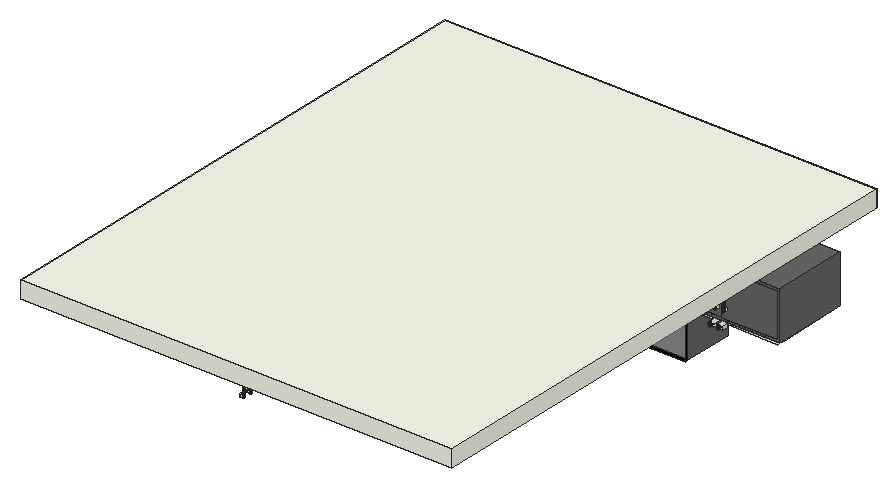
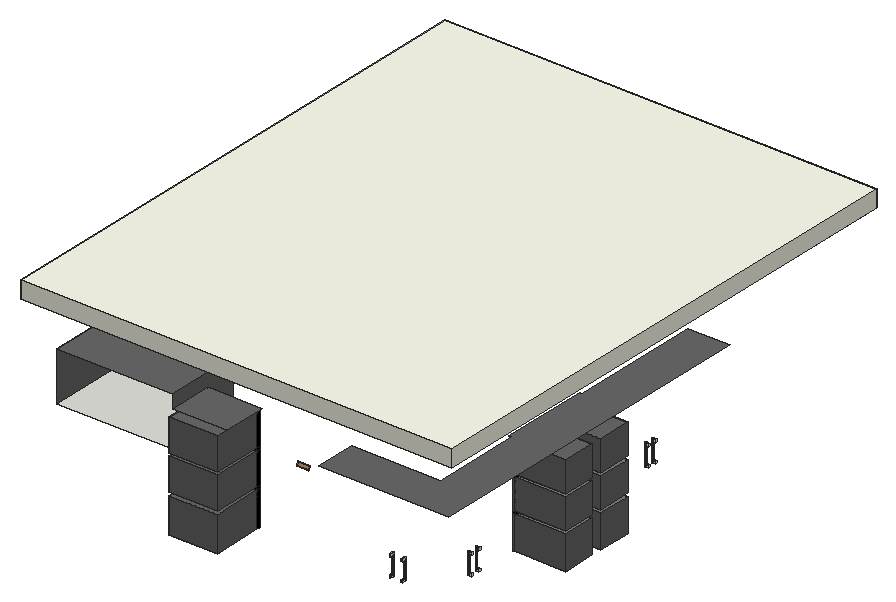
# SketchUp Ruby script. Lengths in inches.
U = 1.inch
M = Sketchup.active_model
def pt(a) = Geom::Point3d.new(a.map { |v| v * U })
def face(e, loops, mat)
  f = e.add_face(loops[0].map { |a| pt(a) })
  loops[1..].each { |l| e.add_face(l.map { |a| pt(a) }).erase! }
  f.material = f.back_material = mat if mat
  f
end
# faces: each face lists its corners as indices into pts; further lists are holes
def faces(e, pts, list, mat = nil) = list.each { |f| face(e, (f[0].is_a?(Array) ? f : [f]).map { |l| l.map { |i| pts[i] } }, mat) }
# xy, xz, yz: faces in a plane at the given z, y or x. An outline is a flat list of corners, or four numbers for a rectangle; further outlines are holes
def ring(l) = l.size == 4 ? [[l[0], l[1]], [l[2], l[1]], [l[2], l[3]], [l[0], l[3]]] : l.each_slice(2).to_a
def flat(e, list, mat, &to3) = list.each { |f| face(e, (f[0].is_a?(Array) ? f : [f]).map { |l| ring(l).map { |u, v| to3.(u, v) } }, mat) }
def xy(e, z, list, mat = nil) = flat(e, list, mat) { |x, y| [x, y, z] }
def xz(e, y, list, mat = nil) = flat(e, list, mat) { |x, z| [x, y, z] }
def yz(e, x, list, mat = nil) = flat(e, list, mat) { |y, z| [x, y, z] }
def lines(e, pts, list) = list.each { |a, b| e.add_line(pt(pts[a]), pt(pts[b])) }
# prism: a flat outline (further loops are holes) pulled along v
def prism(e, loops, v, mat = nil)
  f = face(e, loops, mat); d = Geom::Vector3d.new(v.map { |x| x * U })
  f.pushpull(f.normal.samedirection?(d) ? d.length : -d.length)
end
def box(e, o, s, mat = nil) = prism(e, [[o, [o[0] + s[0], o[1], o[2]], [o[0] + s[0], o[1] + s[1], o[2]], [o[0], o[1] + s[1], o[2]]]], [0, 0, s[2]], mat)
def at(x, y, z, deg = 0) = Geom::Transformation.translation(pt([x, y, z])) * Geom::Transformation.rotation(ORIGIN, Z_AXIS, deg.degrees)
def axes(o, x, y, z) = Geom::Transformation.new([*x, 0, *y, 0, *z, 0, *pt(o).to_a, 1])
def part(name) = M.definitions.add(name)
# library, detail: a bought-in or finely detailed component or shape, given as its bounding box
def library(name, o, s) = part(name).tap { |d| box(d.entities, o, s) }
def detail(e, o, s) = box(e.add_group.entities, o, s)
def put(e, d, t, mat = nil) = e.add_instance(d, t).tap { |i| i.material = mat if mat }
def group(e, t, mat = nil) = e.add_group.tap { |g| g.transformation = t; g.material = mat if mat }.entities
root = M.entities
M.materials.add("[0053_Ivory]").color = [255, 255, 240]
M.materials.add("[0128_White]").color = [255, 255, 255]
M.materials.add("[0133_Gray]").color = [128, 128, 128]
M.materials.add("[0134_DimGray]").color = [105, 105, 105]
M.materials.add("[0137_Black]").color = [0, 0, 0]
M.materials.add("[Translucent Glass Blue]").color = [165, 167, 171]
M.materials["[Translucent Glass Blue]"].alpha = 0.5
c1 = part("Bar")
prism(c1.entities,[[[0,0.49,0.31],[0,0.5,0.25],[0,0.49,0.19],[0,0.47,0.125],[0,0.43,0.07],[0,0.375,0.03],[0,0.31,0.01],[0,0.25,0],[0,0.19,0.01],[0,0.125,0.03],[0,0.07,0.07],[0,0.03,0.125],[0,0.01,0.19],[0,0,0.25],[0,0.01,0.31],[0,0.03,0.375],[0,0.07,0.43],[0,0.125,0.47],[0,0.19,0.49],[0,0.25,0.5],[0,0.31,0.49],[0,0.375,0.47],[0,0.43,0.43],[0,0.47,0.375]]],[11.5,0,0],"[0128_White]")
c2 = part("End")
xy(c2.entities,0,[[0,0.25,0.875,1.5]],"[0128_White]")
xy(c2.entities,0.5,[[0,0.25,0.875,1.5]],"[0128_White]")
xz(c2.entities,1.5,[[0,0,0.875,0.5]],"[0128_White]")
yz(c2.entities,0,[[0.25,0,0.19,0.01,0.125,0.03,0.07,0.07,0.03,0.125,0.01,0.19,0,0.25,0.01,0.31,0.03,0.375,0.07,0.43,0.125,0.47,0.19,0.49,0.25,0.5,1.5,0.5,1.5,0]],"[0128_White]")
yz(c2.entities,0.25,[[0.25,0,0.31,0.01,0.375,0.03,0.43,0.07,0.47,0.125,0.49,0.19,0.5,0.25,0.49,0.31,0.47,0.375,0.43,0.43,0.375,0.47,0.31,0.49,0.25,0.5,0.19,0.49,0.125,0.47,0.07,0.43,0.03,0.375,0.01,0.31,0,0.25,0.01,0.19,0.03,0.125,0.07,0.07,0.125,0.03,0.19,0.01]],"[0128_White]")
yz(c2.entities,0.875,[[0.25,0,1.5,0,1.5,0.5,0.25,0.5,0.31,0.49,0.375,0.47,0.43,0.43,0.47,0.375,0.49,0.31,0.5,0.25,0.49,0.19,0.47,0.125,0.43,0.07,0.375,0.03,0.31,0.01]],"[0128_White]")
p = [[0.25,0.125,0.03],[0,0.125,0.03],[0,0.19,0.01],[0.25,0.19,0.01],[0.25,0.07,0.07],[0,0.07,0.07],
  [0,0.25,0],[0.25,0.25,0],[0.875,0.25,0],[0.875,0.31,0.01],[0.25,0.31,0.01],[0.875,0.375,0.03],
  [0.25,0.375,0.03],[0.875,0.43,0.07],[0.25,0.43,0.07],[0.25,0.01,0.19],[0,0.01,0.19],[0,0.03,0.125],
  [0.25,0.03,0.125],[0.875,0.47,0.125],[0.25,0.47,0.125],[0.875,0.49,0.19],[0.25,0.49,0.19],[0.25,0.01,0.31],
  [0,0.01,0.31],[0,0,0.25],[0.25,0,0.25],[0.875,0.5,0.25],[0.25,0.5,0.25],[0.875,0.49,0.31],
  [0.25,0.49,0.31],[0.25,0.03,0.375],[0,0.03,0.375],[0.875,0.47,0.375],[0.25,0.47,0.375],[0.25,0.07,0.43],
  [0,0.07,0.43],[0.25,0.125,0.47],[0,0.125,0.47],[0.875,0.43,0.43],[0.25,0.43,0.43],[0.875,0.375,0.47],
  [0.25,0.375,0.47],[0.25,0.19,0.49],[0,0.19,0.49],[0.25,0.25,0.5],[0,0.25,0.5],[0.875,0.31,0.49],
  [0.875,0.25,0.5],[0.25,0.31,0.49]]
faces(c2.entities,p,[[0,1,2,3],[4,5,1,0],[3,2,6,7],[8,9,10,7],[9,11,12,10],[11,13,14,12],[15,16,17,18],[18,17,5,4],
  [13,19,20,14],[19,21,22,20],[23,24,25,26],[26,25,16,15],[21,27,28,22],[27,29,30,28],[31,32,24,23],[29,33,34,30],
  [35,36,32,31],[37,38,36,35],[33,39,40,34],[39,41,42,40],[43,44,38,37],[45,46,44,43],[47,48,45,49],[41,47,49,42]],"[0128_White]")
c3 = part("Drawer Pull\#2")
put(c3.entities,c1,axes([0.25,0,0],[0.63,0,0],[0,1,0],[0,0,1]))
put(c3.entities,c2,at(0,0,0))
put(c3.entities,c2,axes([7.74,0,0],[-1,0,0],[0,1,0],[0,0,1]),"[0128_White]")
c4 = library("-   0   +",[0.16,0,-0.06],[4.7,0.79,0.2])
xy(root,67,[[86.34,172,103.87,190]],"[0134_DimGray]")
xy(root,67,[[86.34,171,103.87,172]],"[0137_Black]")
xy(root,68,[[2,110,20.5,122],[20.5,110,21,122],[2,126,20.5,138],[20.5,126,21,138]],"[0134_DimGray]")
xy(root,79.67,[[86.34,172,103.87,190]],"[0134_DimGray]")
xy(root,80,[[2,110,20,122],[2,126,20,138]],"[0133_Gray]")
xy(root,80,[[20,110,20.5,122],[20,126,20.5,138]],"[0137_Black]")
xy(root,80.67,[[86.34,172,103.87,190]],"[0134_DimGray]")
xy(root,81,[[2,110,20,122],[2,126,20,138]],"[0134_DimGray]")
xy(root,81,[[20,110,20.5,122],[20,126,20.5,138]],"[0137_Black]")
xy(root,91.99,[[123.37,157.01,125.37,158.94],[126.37,157.01,128.37,158.94]])
xy(root,92,[[2,110,20,122],[2,126,20,138]],"[0133_Gray]")
xy(root,92,[[20,110,20.5,122],[20,126,20.5,138]],"[0137_Black]")
xy(root,92.33,[[86.34,172,103.87,190]],"[0134_DimGray]")
xy(root,92.99,[[123.37,157.11,125.37,157.11,125.37,159.6875,104.87,159.6875,104.87,158.94,123.37,158.94],[126.37,157.11,128.37,157.11,128.37,158.94,146.87,158.94,146.87,159.6875,126.37,159.6875],[104.87,159.6875,125.37,160.87],[104.87,161.84,104.87,187,146.87,187,146.87,161.85,125.37,161.85,125.37,161.84]])
xy(root,92.99,[[125.37,159.6875,125.37,160.87,104.87,160.87,104.87,161.84,125.37,161.84,125.37,161.85,146.87,161.85,146.87,160.88,126.37,160.88,126.37,159.6875],[126.37,159.6875,146.87,160.88]],"[0053_Ivory]")
xy(root,93,[[2,110,20,122],[2,126,20,138]],"[0134_DimGray]")
xy(root,93,[[20,110,20.5,122],[20,126,20.5,138]],"[0137_Black]")
xy(root,93.33,[[86.34,172,103.87,190]],"[0134_DimGray]")
xy(root,104,[[2,110,20.5,122],[20.5,110,21,122],[2,126,20.5,138],[20.5,126,21,138]],"[0134_DimGray]")
xy(root,105,[[86.34,172,103.87,190]],"[0134_DimGray]")
xy(root,105,[[86.34,171,103.87,172]],"[0137_Black]")
xy(root,106,[[5,60,20,60,20,108,21,108,21,140,20,140,20,172,52,172,52,187,5,187],[85.34,171,104.87,187]],"[0134_DimGray]")
xy(root,110.79,[[104.87,159.6875,146.87,187]],"[0134_DimGray]")
xy(root,126,[[0,0,0,192,156,192,156,187,5,187,5,0],[[5,0,156,187],[29,24,132,163]]],"[0053_Ivory]")
xy(root,130,[[29,24,132,163]],"[0053_Ivory]")
xy(root,132,[[0,0,156,192]],"[0053_Ivory]")
xz(root,0,[[0,126,156,132]],"[0053_Ivory]")
xz(root,24,[[29,126,132,130]],"[0053_Ivory]")
xz(root,110,[[2,68,20.5,80],[20.5,68,21,80],[2,81,20.5,92],[20.5,81,21,92],[2,93,20.5,104],
  [20.5,93,21,104]],"[0134_DimGray]")
xz(root,110,[[20,80,21,81],[20,92,21,93]],"[0137_Black]")
xz(root,122,[[2,68,20.5,80],[20.5,68,21,80],[2,81,20.5,92],[20.5,81,21,92],[2,93,20.5,104],
  [20.5,93,21,104]],"[0134_DimGray]")
xz(root,122,[[20,80,21,81],[20,92,21,93]],"[0137_Black]")
xz(root,126,[[2,68,20.5,80],[20.5,68,21,80],[2,81,20.5,92],[20.5,81,21,92],[2,93,20.5,104],
  [20.5,93,21,104]],"[0134_DimGray]")
xz(root,126,[[20,80,21,81],[20,92,21,93]],"[0137_Black]")
xz(root,138,[[2,68,20.5,80],[20.5,68,21,80],[2,81,20.5,92],[20.5,81,21,92],[2,93,20.5,104],
  [20.5,93,21,104]],"[0134_DimGray]")
xz(root,138,[[20,80,21,81],[20,92,21,93]],"[0137_Black]")
xz(root,159.6875,[[[104.87,92.99,146.87,110.79],[105.87,93.99,145.87,109.79]],[105.87,93.99,125.87,109.79],[125.87,93.99,145.87,109.79]],"[0134_DimGray]")
xz(root,163,[[29,126,132,130]],"[0053_Ivory]")
xz(root,172,[[86.34,79.67,103.87,80.67],[86.34,92.33,103.87,93.33]],"[0137_Black]")
xz(root,172,[[86.34,67,103.87,79.67],[86.34,80.67,103.87,92.33],[86.34,93.33,103.87,105]],"[Translucent Glass Blue]")
xz(root,190,[[86.34,67,103.87,79.67],[86.34,80.67,103.87,92.33],[86.34,93.33,103.87,105]],"[0134_DimGray]")
xz(root,192,[[0,126,156,132]],"[0053_Ivory]")
yz(root,0,[[0,126,192,132]],"[0053_Ivory]")
yz(root,2,[[110,68,122,80],[126,68,138,80],[110,81,122,92],[126,81,138,92],[110,93,122,104],
  [126,93,138,104]],"[0134_DimGray]")
yz(root,20,[[110,80,122,81],[126,80,138,81],[110,92,122,93],[126,92,138,93]],"[0137_Black]")
yz(root,20.5,[[110,68,122,80],[126,68,138,80],[110,81,122,92],[126,81,138,92],[110,93,122,104],
  [126,93,138,104]],"[Translucent Glass Blue]")
yz(root,29,[[24,126,163,130]],"[0053_Ivory]")
yz(root,86.34,[[172,67,190,79.67],[172,80.67,190,92.33],[172,93.33,190,105]],"[0134_DimGray]")
yz(root,86.34,[[171,67,172,79.67],[171,79.67,172,80.67],[171,80.67,172,92.33],[171,92.33,172,93.33],[171,93.33,172,105]],"[0137_Black]")
yz(root,103.87,[[172,67,190,79.67],[172,80.67,190,92.33],[172,93.33,190,105]],"[0134_DimGray]")
yz(root,103.87,[[171,67,172,79.67],[171,79.67,172,80.67],[171,80.67,172,92.33],[171,92.33,172,93.33],[171,93.33,172,105]],"[0137_Black]")
yz(root,104.87,[[159.6875,92.99,159.6875,110.79,187,110.79,187,106,171,106,171,92.99]],"[0134_DimGray]")
yz(root,123.37,[[157.11,91.99,158.94,92.99]])
yz(root,128.37,[[157.11,91.99,158.94,92.99]])
yz(root,132,[[24,126,163,130]],"[0053_Ivory]")
yz(root,146.87,[[159.6875,92.99,187,110.79]],"[0134_DimGray]")
yz(root,156,[[0,126,192,132]],"[0053_Ivory]")
p = [[124.37,156.14,91.99],[124.625,156.17,92.25],[124.11,156.17,92.25],[127.11,156.17,92.25],[127.37,156.14,91.99],[127.625,156.17,92.25],
  [124.87,156.27,92.49],[123.87,156.27,92.49],[126.87,156.27,92.49],[127.87,156.27,92.49],[125.07,156.42,92.7],[123.66,156.42,92.7],
  [126.66,156.42,92.7],[128.07,156.42,92.7],[105.35,161.23,92.51],[105.3,161.11,92.56],[124.93,161.11,92.56],[124.88,161.23,92.51],
  [126.85,161.24,92.51],[126.8,161.12,92.5625],[146.43,161.12,92.5625],[146.38,161.24,92.51],[105.37,161.36,92.49],[124.86,161.36,92.49],
  [126.87,161.36,92.49],[146.37,161.36,92.49],[105.35,161.48,92.51],[124.88,161.48,92.51],[126.85,161.49,92.51],[146.38,161.49,92.51],
  [105.3,161.6,92.56],[124.93,161.6,92.56],[126.8,161.6,92.5625],[146.43,161.6,92.5625],[105.22,161.01,92.64],[105.12,160.9375,92.74],
  [125.11,160.9375,92.74],[125.01,161.01,92.64],[126.72,161.02,92.64],[126.62,160.94,92.74],[146.62,160.94,92.74],[146.51,161.02,92.64],
  [105.22,161.7,92.64],[125.01,161.7,92.64],[126.72,161.7,92.64],[146.51,161.7,92.64],[105.12,161.78,92.74],[125.11,161.78,92.74],
  [126.62,161.78,92.74],[146.62,161.78,92.74],[125.23,156.62,92.86],[123.5,156.62,92.86],[126.5,156.62,92.86],[128.23,156.62,92.86],
  [105,160.89,92.86],[125.24,160.89,92.86],[126.5,160.89,92.86],[146.74,160.89,92.86],[105,161.83,92.86],[125.24,161.83,92.86],
  [126.5,161.83,92.86],[146.74,161.83,92.86],[125.33,156.86,92.96],[123.4,156.86,92.96],[126.4,156.86,92.96],[128.33,156.86,92.96],
  [104.87,160.87,92.99],[125.37,160.87,92.99],[126.37,160.88,92.99],[146.87,160.88,92.99],[104.87,161.84,92.99],[125.37,161.84,92.99],
  [126.37,161.85,92.99],[146.87,161.85,92.99],[125.37,157.11,92.99],[123.37,157.11,92.99],[126.37,157.11,92.99],[128.37,157.11,92.99]]
faces(root,p,[[0,1,2],[3,4,5],[1,6,7,2],[8,3,5,9],[6,10,11,7],[12,8,9,13],[10,50,51,11],[52,12,13,53],
  [50,62,63,51],[64,52,53,65],[62,74,75,63],[76,64,65,77]])
faces(root,p,[[14,15,16,17],[18,19,20,21],[22,14,17,23],[24,18,21,25],[26,22,23,27],[28,24,25,29],[30,26,27,31],[32,28,29,33],
  [34,35,36,37],[38,39,40,41],[15,34,37,16],[19,38,41,20],[42,30,31,43],[44,32,33,45],[46,42,43,47],[48,44,45,49],
  [35,54,55,36],[39,56,57,40],[58,46,47,59],[60,48,49,61],[54,66,67,55],[56,68,69,57],[70,58,59,71],[72,60,61,73]],"[0137_Black]")
put(root,c3,axes([33.72,170.5,75.83],[0,0,-1],[0,1,0],[1,0,0]),"[0128_White]")
put(root,c3,axes([37.97,170.5,75.83],[0,0,-1],[0,1,0],[1,0,0]),"[0128_White]")
put(root,c3,axes([21.5,74.21,76.5],[0,0,-1],[-1,0,0],[0,1,0]),"[0128_White]")
put(root,c3,axes([21.5,77.34,76.5],[0,0,-1],[-1,0,0],[0,1,0]),"[0128_White]")
put(root,c3,axes([21.5,90.09,76.5],[0,0,-1],[-1,0,0],[0,1,0]),"[0128_White]")
put(root,c3,axes([21.5,93.02,76.5],[0,0,-1],[-1,0,0],[0,1,0]),"[0128_White]")
put(root,c3,axes([21.5,154.02,76.5],[0,0,-1],[-1,0,0],[0,1,0]),"[0128_White]")
put(root,c3,axes([21.5,157.4,76.5],[0,0,-1],[-1,0,0],[0,1,0]),"[0128_White]")
put(root,c4,axes([67.07,172.55,93.0625],[0.90257,0,0],[0,-0.48894,1.48201],[0,-0.84686,-0.85564]))
put(root,c3,axes([124.26,158.1875,104.53],[0,0,-1],[0,1,0],[1,0,0]),"[0128_White]")
put(root,c3,axes([127.33,158.1875,104.53],[0,0,-1],[0,1,0],[1,0,0]),"[0128_White]")
